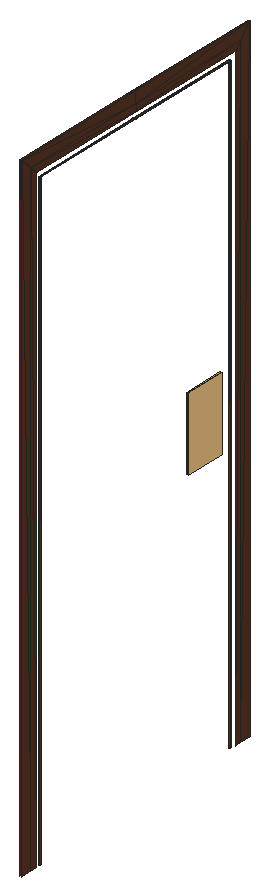
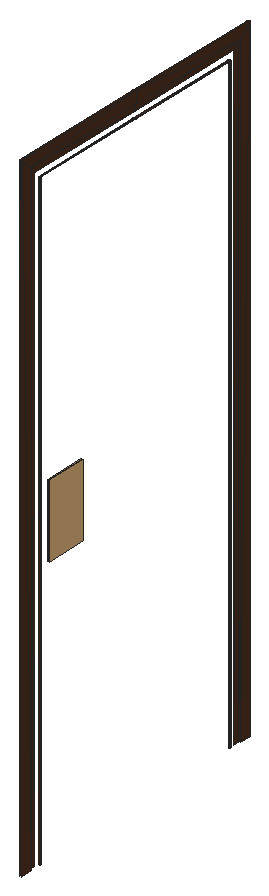
# SketchUp Ruby script. Lengths in inches.
U = 1.inch
M = Sketchup.active_model
def pt(a) = Geom::Point3d.new(a.map { |v| v * U })
def face(e, loops, mat)
  f = e.add_face(loops[0].map { |a| pt(a) })
  loops[1..].each { |l| e.add_face(l.map { |a| pt(a) }).erase! }
  f.material = f.back_material = mat if mat
  f
end
# faces: each face lists its corners as indices into pts; further lists are holes
def faces(e, pts, list, mat = nil) = list.each { |f| face(e, (f[0].is_a?(Array) ? f : [f]).map { |l| l.map { |i| pts[i] } }, mat) }
# xy, xz, yz: faces in a plane at the given z, y or x. An outline is a flat list of corners, or four numbers for a rectangle; further outlines are holes
def ring(l) = l.size == 4 ? [[l[0], l[1]], [l[2], l[1]], [l[2], l[3]], [l[0], l[3]]] : l.each_slice(2).to_a
def flat(e, list, mat, &to3) = list.each { |f| face(e, (f[0].is_a?(Array) ? f : [f]).map { |l| ring(l).map { |u, v| to3.(u, v) } }, mat) }
def xy(e, z, list, mat = nil) = flat(e, list, mat) { |x, y| [x, y, z] }
def xz(e, y, list, mat = nil) = flat(e, list, mat) { |x, z| [x, y, z] }
def yz(e, x, list, mat = nil) = flat(e, list, mat) { |y, z| [x, y, z] }
def lines(e, pts, list) = list.each { |a, b| e.add_line(pt(pts[a]), pt(pts[b])) }
# prism: a flat outline (further loops are holes) pulled along v
def prism(e, loops, v, mat = nil)
  f = face(e, loops, mat); d = Geom::Vector3d.new(v.map { |x| x * U })
  f.pushpull(f.normal.samedirection?(d) ? d.length : -d.length)
end
def box(e, o, s, mat = nil) = prism(e, [[o, [o[0] + s[0], o[1], o[2]], [o[0] + s[0], o[1] + s[1], o[2]], [o[0], o[1] + s[1], o[2]]]], [0, 0, s[2]], mat)
def at(x, y, z, deg = 0) = Geom::Transformation.translation(pt([x, y, z])) * Geom::Transformation.rotation(ORIGIN, Z_AXIS, deg.degrees)
def axes(o, x, y, z) = Geom::Transformation.new([*x, 0, *y, 0, *z, 0, *pt(o).to_a, 1])
def part(name) = M.definitions.add(name)
# library, detail: a bought-in or finely detailed component or shape, given as its bounding box
def library(name, o, s) = part(name).tap { |d| box(d.entities, o, s) }
def detail(e, o, s) = box(e.add_group.entities, o, s)
def put(e, d, t, mat = nil) = e.add_instance(d, t).tap { |i| i.material = mat if mat }
def group(e, t, mat = nil) = e.add_group.tap { |g| g.transformation = t; g.material = mat if mat }.entities
root = M.entities
M.materials.add("Material \#0").color = [86, 53, 35]
M.materials.add("Material \#1").color = [140, 140, 140]
c1 = part("3DGeom~21_Defintion")
xy(c1.entities,73.08,[[-976.3,-241.71,23.7,-241.71,-976.3,-223.46],[23.7,-241.71,5.45,-223.46,-976.3,-223.46],[23.7,-241.71,23.7,0,5.45,-223.46],[5.45,-223.46,23.7,0,5.45,0],[23.7,0,23.7,241.71,5.45,223.46],
  [5.45,0,23.7,0,5.45,223.46],[-976.3,223.46,23.7,241.71,-976.3,241.71],[-976.3,223.46,5.45,223.46,23.7,241.71]],"Material \#0")
c2 = part("3DGeom~22_Defintion")
xz(c2.entities,-210.625,[[-1016.13,2.47,-1016.13,9.96,-16.28,2.47],[-16.28,2.47,-1016.13,9.96,-16.28,9.96],[-1016.13,9.96,-1016.13,51.7,-16.28,51.7],[-1016.13,9.96,-16.28,51.7,-16.28,9.96],[-1016.13,51.7,-1016.13,72.71,-16.28,51.7]],"Material \#0")
xz(c2.entities,210.625,[[-1016.13,2.47,-16.28,2.47,-1016.13,9.96],[-16.28,2.47,-16.28,9.96,-1016.13,9.96],[-1016.13,9.96,-16.28,51.7,-1016.13,51.7],[-1016.13,9.96,-16.28,9.96,-16.28,51.7],[-1016.13,51.7,-16.28,51.7,-1016.13,72.71]],"Material \#0")
yz(c2.entities,-16.28,[[-210.625,2.47,-210.625,9.96,0,9.96],[-210.625,2.47,0,9.96,0,2.47],[0,2.47,0,9.96,210.625,2.47],[210.625,2.47,0,9.96,210.625,9.96],[-210.625,9.96,-210.625,51.7,0,51.7],
  [-210.625,9.96,0,51.7,0,9.96],[0,9.96,0,51.7,210.625,9.96],[210.625,9.96,0,51.7,210.625,51.7],[-210.625,51.7,0,72.71,0,51.7],[0,51.7,0,72.71,210.625,51.7]],"Material \#0")
p = [[-1016.13,-210.625,72.71],[-16.13,-210.77,73.09],[-16.28,-210.625,51.7],[-16.28,-210.625,51.7],[-16.13,-210.77,73.09],[-16.28,0,72.71],
  [-16.13,210.77,73.09],[-16.28,210.625,51.7],[-16.28,210.625,51.7],[-16.13,210.77,73.09],[-1016.13,210.625,72.71]]
faces(c2.entities,p,[[0,1,2],[3,4,5],[5,6,7],[8,9,10]],"Material \#0")
c3 = part("3DGeom~20_Defintion")
xy(c3.entities,0,[[-976.3,-241.71,-976.3,-223.46,23.7,-241.71],[23.7,-241.71,-976.3,-223.46,5.45,-223.46],[23.7,-241.71,5.45,-223.46,5.45,0],[23.7,-241.71,5.45,0,23.7,0],[-976.3,-223.46,-976.3,-211.85,5.45,-223.46],
  [5.45,-223.46,-976.3,-211.85,-6.16,-211.85],[5.45,-223.46,-6.16,-211.85,-6.16,0],[5.45,-223.46,-6.16,0,5.45,0],[-6.16,0,-6.16,211.85,5.45,223.46],[-6.16,0,5.45,223.46,5.45,0],
  [5.45,0,23.7,241.71,23.7,0],[5.45,0,5.45,223.46,23.7,241.71],[-976.3,211.85,-976.3,223.46,5.45,223.46],[-976.3,211.85,5.45,223.46,-6.16,211.85],[-976.3,223.46,-976.3,241.71,23.7,241.71],
  [-976.3,223.46,23.7,241.71,5.45,223.46]],"Material \#0")
c4 = part("3DGeom~18_Defintion")
xz(c4.entities,-241.71,[[-976.3,0,23.7,0,23.7,7.58],[-976.3,0,23.7,7.58,-976.3,7.58]],"Material \#0")
xz(c4.entities,241.71,[[-976.3,0,-976.3,7.58,23.7,7.58],[-976.3,0,23.7,7.58,23.7,0]],"Material \#0")
yz(c4.entities,23.7,[[-241.71,0,0,0,-241.71,7.58],[0,0,0,7.58,-241.71,7.58],[0,0,241.71,0,241.71,7.58],[0,0,241.71,7.58,0,7.58]],"Material \#0")
c5 = library("3DGeom~3_Defintion",[-83.33,-500,-350],[620.1,1000,533.33])
yz(root,362.57,[[201.19,43.83,201.125,43.95,201.11,43.95],[201.11,43.95,201.07,44.09,201.06,44.08],[201.11,43.95,201.125,43.95,201.07,44.09],[201.06,44.08,201.07,44.09,201.03,44.23]],"Material \#1")
yz(root,362.69,[[201.4,43.64,201.29,43.72,201.3,43.73],[201.4,43.64,201.3,43.73,201.41,43.65],[201.29,43.72,201.19,43.83,201.2,43.83],[201.29,43.72,201.2,43.83,201.3,43.73],[201.19,43.83,201.11,43.95,201.125,43.95],
  [201.19,43.83,201.125,43.95,201.2,43.83],[201.11,43.95,201.06,44.08,201.07,44.09],[201.11,43.95,201.07,44.09,201.125,43.95],[201.06,44.08,201.02,44.23,201.03,44.23],[201.06,44.08,201.03,44.23,201.07,44.09],
  [201.02,44.23,201.01,44.39,201.02,44.39],[201.02,44.23,201.02,44.39,201.03,44.23],[201.01,44.39,201.01,54.24,201.02,54.24],[201.01,44.39,201.02,52.11,201.02,44.39],[201.01,44.39,201.02,54.24,201.02,52.11]],"Material \#1")
put(root,c1,axes([362.93,185.06,101.58],[0,0,0.10405],[0,-0.09548,0],[-0.00434,0,0]),"Material \#0")
put(root,c2,axes([362.93,185.06,101.58],[0,0,0.09997],[0,-0.09173,0],[-0.00417,0,0]),"Material \#0")
put(root,c3,axes([362.93,185.06,101.58],[0,0,0.10405],[0,-0.09548,0],[-0.00434,0,0]),"Material \#0")
put(root,c4,axes([362.93,185.06,101.58],[0,0,0.10405],[0,-0.09548,0],[-0.00434,0,0]),"Material \#0")
put(root,c5,axes([362.67,201.8,49.3125],[0,-0.01086,0],[0,0,0.01184],[0.00049,0,0]),"Material \#1")
